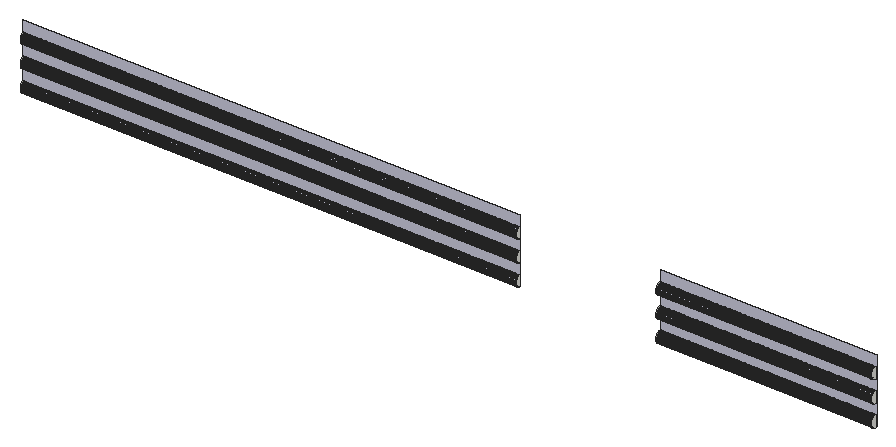
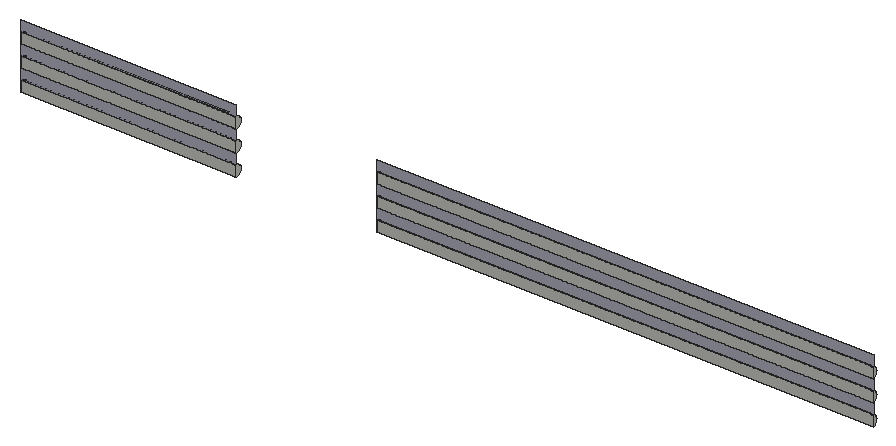
# SketchUp Ruby script. Lengths in millimetres.
U = 1.mm
M = Sketchup.active_model
def pt(a) = Geom::Point3d.new(a.map { |v| v * U })
def face(e, loops, mat)
  f = e.add_face(loops[0].map { |a| pt(a) })
  loops[1..].each { |l| e.add_face(l.map { |a| pt(a) }).erase! }
  f.material = f.back_material = mat if mat
  f
end
# faces: each face lists its corners as indices into pts; further lists are holes
def faces(e, pts, list, mat = nil) = list.each { |f| face(e, (f[0].is_a?(Array) ? f : [f]).map { |l| l.map { |i| pts[i] } }, mat) }
# xy, xz, yz: faces in a plane at the given z, y or x. An outline is a flat list of corners, or four numbers for a rectangle; further outlines are holes
def ring(l) = l.size == 4 ? [[l[0], l[1]], [l[2], l[1]], [l[2], l[3]], [l[0], l[3]]] : l.each_slice(2).to_a
def flat(e, list, mat, &to3) = list.each { |f| face(e, (f[0].is_a?(Array) ? f : [f]).map { |l| ring(l).map { |u, v| to3.(u, v) } }, mat) }
def xy(e, z, list, mat = nil) = flat(e, list, mat) { |x, y| [x, y, z] }
def xz(e, y, list, mat = nil) = flat(e, list, mat) { |x, z| [x, y, z] }
def yz(e, x, list, mat = nil) = flat(e, list, mat) { |y, z| [x, y, z] }
def lines(e, pts, list) = list.each { |a, b| e.add_line(pt(pts[a]), pt(pts[b])) }
# prism: a flat outline (further loops are holes) pulled along v
def prism(e, loops, v, mat = nil)
  f = face(e, loops, mat); d = Geom::Vector3d.new(v.map { |x| x * U })
  f.pushpull(f.normal.samedirection?(d) ? d.length : -d.length)
end
def box(e, o, s, mat = nil) = prism(e, [[o, [o[0] + s[0], o[1], o[2]], [o[0] + s[0], o[1] + s[1], o[2]], [o[0], o[1] + s[1], o[2]]]], [0, 0, s[2]], mat)
def at(x, y, z, deg = 0) = Geom::Transformation.translation(pt([x, y, z])) * Geom::Transformation.rotation(ORIGIN, Z_AXIS, deg.degrees)
def axes(o, x, y, z) = Geom::Transformation.new([*x, 0, *y, 0, *z, 0, *pt(o).to_a, 1])
def part(name) = M.definitions.add(name)
# library, detail: a bought-in or finely detailed component or shape, given as its bounding box
def library(name, o, s) = part(name).tap { |d| box(d.entities, o, s) }
def detail(e, o, s) = box(e.add_group.entities, o, s)
def put(e, d, t, mat = nil) = e.add_instance(d, t).tap { |i| i.material = mat if mat }
def group(e, t, mat = nil) = e.add_group.tap { |g| g.transformation = t; g.material = mat if mat }.entities
root = M.entities
M.materials.add("[0116_Lavender]").color = [197, 197, 214]
xz(root,16548.1,[[11038.5,12969.9,25059.3,13274.7],[29021.7,12969.9,35117.7,13274.7],[11038.5,13579.5,25059.3,13884.3],[29021.7,13579.5,35117.7,13884.3],[11038.5,14189.1,25059.3,14493.9],
  [29021.7,14189.1,35117.7,14493.9]])
xz(root,16548.1,[[11038.5,13274.7,25059.3,13579.5],[29021.7,13274.7,35117.7,13579.5],[11038.5,13884.3,25059.3,14189.1],[29021.7,13884.3,35117.7,14189.1],[11038.5,14493.9,25059.3,14798.7],
  [29021.7,14493.9,35117.7,14798.7]],"[0116_Lavender]")
yz(root,11038.5,[[16548.1,12969.9,16536.2,12975.2,16524.8,12981.5,16514,12988.6,16503.7,12996.6,16494.1,13005.4,16485.2,13014.9,16477.1,13025,16469.8,13035.8,16463.4,13047.1,16458,13058.9,16453.4,13071.1,16449.9,13083.6,16447.3,13096.4,16445.8,13109.3,16445.3,13122.3,16445.8,13135.3,16447.3,13148.2,16449.9,13160.9,16453.4,13173.4,16458,13185.6,16463.4,13197.4,16469.8,13208.7,16477.1,13219.5,16485.2,13229.7,16494.1,13239.2,16503.7,13248,16514,13255.9,16524.8,13263.1,16536.2,13269.3,16548.1,13274.7],[16548.1,13579.5,16536.2,13584.8,16524.8,13591.1,16514,13598.2,16503.7,13606.2,16494.1,13615,16485.2,13624.5,16477.1,13634.6,16469.8,13645.4,16463.4,13656.7,16458,13668.5,16453.4,13680.7,16449.9,13693.2,16447.3,13706,16445.8,13718.9,16445.3,13731.9,16445.8,13744.9,16447.3,13757.8,16449.9,13770.5,16453.4,13783,16458,13795.2,16463.4,13807,16469.8,13818.3,16477.1,13829.1,16485.2,13839.3,16494.1,13848.8,16503.7,13857.6,16514,13865.5,16524.8,13872.7,16536.2,13878.9,16548.1,13884.3],[16548.1,14189.1,16536.2,14194.4,16524.8,14200.7,16514,14207.8,16503.7,14215.8,16494.1,14224.6,16485.2,14234.1,16477.1,14244.2,16469.8,14255,16463.4,14266.3,16458,14278.1,16453.4,14290.3,16449.9,14302.8,16447.3,14315.6,16445.8,14328.5,16445.3,14341.5,16445.8,14354.5,16447.3,14367.4,16449.9,14380.1,16453.4,14392.6,16458,14404.8,16463.4,14416.6,16469.8,14427.9,16477.1,14438.7,16485.2,14448.9,16494.1,14458.4,16503.7,14467.2,16514,14475.1,16524.8,14482.3,16536.2,14488.5,16548.1,14493.9]])
yz(root,25059.3,[[16548.1,12969.9,16548.1,13274.7,16536.2,13269.3,16524.8,13263.1,16514,13255.9,16503.7,13248,16494.1,13239.2,16485.2,13229.7,16477.1,13219.5,16469.8,13208.7,16463.4,13197.4,16458,13185.6,16453.4,13173.4,16449.9,13160.9,16447.3,13148.2,16445.8,13135.3,16445.3,13122.3,16445.8,13109.3,16447.3,13096.4,16449.9,13083.6,16453.4,13071.1,16458,13058.9,16463.4,13047.1,16469.8,13035.8,16477.1,13025,16485.2,13014.9,16494.1,13005.4,16503.7,12996.6,16514,12988.6,16524.8,12981.5,16536.2,12975.2],[16548.1,13579.5,16548.1,13884.3,16536.2,13878.9,16524.8,13872.7,16514,13865.5,16503.7,13857.6,16494.1,13848.8,16485.2,13839.3,16477.1,13829.1,16469.8,13818.3,16463.4,13807,16458,13795.2,16453.4,13783,16449.9,13770.5,16447.3,13757.8,16445.8,13744.9,16445.3,13731.9,16445.8,13718.9,16447.3,13706,16449.9,13693.2,16453.4,13680.7,16458,13668.5,16463.4,13656.7,16469.8,13645.4,16477.1,13634.6,16485.2,13624.5,16494.1,13615,16503.7,13606.2,16514,13598.2,16524.8,13591.1,16536.2,13584.8],[16548.1,14189.1,16548.1,14493.9,16536.2,14488.5,16524.8,14482.3,16514,14475.1,16503.7,14467.2,16494.1,14458.4,16485.2,14448.9,16477.1,14438.7,16469.8,14427.9,16463.4,14416.6,16458,14404.8,16453.4,14392.6,16449.9,14380.1,16447.3,14367.4,16445.8,14354.5,16445.3,14341.5,16445.8,14328.5,16447.3,14315.6,16449.9,14302.8,16453.4,14290.3,16458,14278.1,16463.4,14266.3,16469.8,14255,16477.1,14244.2,16485.2,14234.1,16494.1,14224.6,16503.7,14215.8,16514,14207.8,16524.8,14200.7,16536.2,14194.4]])
yz(root,29021.7,[[16548.1,12969.9,16540.1,12970.1,16532.2,12970.7,16524.3,12971.8,16516.4,12973.2,16508.7,12975.1,16501,12977.3,16493.5,12980,16486.1,12983.1,16478.9,12986.5,16471.9,12990.3,16465.1,12994.5,16458.5,12999,16452.2,13003.8,16446.1,13009,16440.3,13014.5,16434.8,13020.3,16429.7,13026.4,16424.8,13032.7,16420.3,13039.3,16416.1,13046.1,16412.3,13053.1,16408.9,13060.3,16405.8,13067.7,16403.2,13075.2,16400.9,13082.8,16399,13090.6,16397.6,13098.4,16396.5,13106.3,16395.9,13114.3,16395.7,13122.3,16395.9,13130.3,16396.5,13138.2,16397.6,13146.1,16399,13154,16400.9,13161.7,16403.2,13169.4,16405.8,13176.9,16408.9,13184.3,16412.3,13191.5,16416.1,13198.5,16420.3,13205.3,16424.8,13211.9,16429.7,13218.2,16434.8,13224.3,16440.3,13230,16446.1,13235.5,16452.2,13240.7,16458.5,13245.6,16465.1,13250.1,16471.9,13254.3,16478.9,13258.1,16486.1,13261.5,16493.5,13264.6,16501,13267.2,16508.7,13269.5,16516.4,13271.3,16524.3,13272.8,16532.2,13273.8,16540.1,13274.5,16548.1,13274.7],[16548.1,13579.5,16540.1,13579.7,16532.2,13580.3,16524.3,13581.4,16516.4,13582.8,16508.7,13584.7,16501,13586.9,16493.5,13589.6,16486.1,13592.7,16478.9,13596.1,16471.9,13599.9,16465.1,13604.1,16458.5,13608.6,16452.2,13613.4,16446.1,13618.6,16440.3,13624.1,16434.8,13629.9,16429.7,13636,16424.8,13642.3,16420.3,13648.9,16416.1,13655.7,16412.3,13662.7,16408.9,13669.9,16405.8,13677.3,16403.2,13684.8,16400.9,13692.4,16399,13700.2,16397.6,13708,16396.5,13715.9,16395.9,13723.9,16395.7,13731.9,16395.9,13739.9,16396.5,13747.8,16397.6,13755.7,16399,13763.6,16400.9,13771.3,16403.2,13779,16405.8,13786.5,16408.9,13793.9,16412.3,13801.1,16416.1,13808.1,16420.3,13814.9,16424.8,13821.5,16429.7,13827.8,16434.8,13833.9,16440.3,13839.6,16446.1,13845.1,16452.2,13850.3,16458.5,13855.2,16465.1,13859.7,16471.9,13863.9,16478.9,13867.7,16486.1,13871.1,16493.5,13874.2,16501,13876.8,16508.7,13879.1,16516.4,13880.9,16524.3,13882.4,16532.2,13883.4,16540.1,13884.1,16548.1,13884.3],[16548.1,14189.1,16540.1,14189.3,16532.2,14189.9,16524.3,14191,16516.4,14192.4,16508.7,14194.3,16501,14196.5,16493.5,14199.2,16486.1,14202.3,16478.9,14205.7,16471.9,14209.5,16465.1,14213.7,16458.5,14218.2,16452.2,14223,16446.1,14228.2,16440.3,14233.7,16434.8,14239.5,16429.7,14245.6,16424.8,14251.9,16420.3,14258.5,16416.1,14265.3,16412.3,14272.3,16408.9,14279.5,16405.8,14286.9,16403.2,14294.4,16400.9,14302,16399,14309.8,16397.6,14317.6,16396.5,14325.5,16395.9,14333.5,16395.7,14341.5,16395.9,14349.5,16396.5,14357.4,16397.6,14365.3,16399,14373.2,16400.9,14380.9,16403.2,14388.6,16405.8,14396.1,16408.9,14403.5,16412.3,14410.7,16416.1,14417.7,16420.3,14424.5,16424.8,14431.1,16429.7,14437.4,16434.8,14443.5,16440.3,14449.2,16446.1,14454.7,16452.2,14459.9,16458.5,14464.8,16465.1,14469.3,16471.9,14473.5,16478.9,14477.3,16486.1,14480.7,16493.5,14483.8,16501,14486.4,16508.7,14488.7,16516.4,14490.5,16524.3,14492,16532.2,14493,16540.1,14493.7,16548.1,14493.9]])
yz(root,35117.7,[[16548.1,12969.9,16548.1,13274.7,16540.1,13274.5,16532.2,13273.8,16524.3,13272.8,16516.4,13271.3,16508.7,13269.5,16501,13267.2,16493.5,13264.6,16486.1,13261.5,16478.9,13258.1,16471.9,13254.3,16465.1,13250.1,16458.5,13245.6,16452.2,13240.7,16446.1,13235.5,16440.3,13230,16434.8,13224.3,16429.7,13218.2,16424.8,13211.9,16420.3,13205.3,16416.1,13198.5,16412.3,13191.5,16408.9,13184.3,16405.8,13176.9,16403.2,13169.4,16400.9,13161.7,16399,13154,16397.6,13146.1,16396.5,13138.2,16395.9,13130.3,16395.7,13122.3,16395.9,13114.3,16396.5,13106.3,16397.6,13098.4,16399,13090.6,16400.9,13082.8,16403.2,13075.2,16405.8,13067.7,16408.9,13060.3,16412.3,13053.1,16416.1,13046.1,16420.3,13039.3,16424.8,13032.7,16429.7,13026.4,16434.8,13020.3,16440.3,13014.5,16446.1,13009,16452.2,13003.8,16458.5,12999,16465.1,12994.5,16471.9,12990.3,16478.9,12986.5,16486.1,12983.1,16493.5,12980,16501,12977.3,16508.7,12975.1,16516.4,12973.2,16524.3,12971.8,16532.2,12970.7,16540.1,12970.1],[16548.1,13579.5,16548.1,13884.3,16540.1,13884.1,16532.2,13883.4,16524.3,13882.4,16516.4,13880.9,16508.7,13879.1,16501,13876.8,16493.5,13874.2,16486.1,13871.1,16478.9,13867.7,16471.9,13863.9,16465.1,13859.7,16458.5,13855.2,16452.2,13850.3,16446.1,13845.1,16440.3,13839.6,16434.8,13833.9,16429.7,13827.8,16424.8,13821.5,16420.3,13814.9,16416.1,13808.1,16412.3,13801.1,16408.9,13793.9,16405.8,13786.5,16403.2,13779,16400.9,13771.3,16399,13763.6,16397.6,13755.7,16396.5,13747.8,16395.9,13739.9,16395.7,13731.9,16395.9,13723.9,16396.5,13715.9,16397.6,13708,16399,13700.2,16400.9,13692.4,16403.2,13684.8,16405.8,13677.3,16408.9,13669.9,16412.3,13662.7,16416.1,13655.7,16420.3,13648.9,16424.8,13642.3,16429.7,13636,16434.8,13629.9,16440.3,13624.1,16446.1,13618.6,16452.2,13613.4,16458.5,13608.6,16465.1,13604.1,16471.9,13599.9,16478.9,13596.1,16486.1,13592.7,16493.5,13589.6,16501,13586.9,16508.7,13584.7,16516.4,13582.8,16524.3,13581.4,16532.2,13580.3,16540.1,13579.7],[16548.1,14189.1,16548.1,14493.9,16540.1,14493.7,16532.2,14493,16524.3,14492,16516.4,14490.5,16508.7,14488.7,16501,14486.4,16493.5,14483.8,16486.1,14480.7,16478.9,14477.3,16471.9,14473.5,16465.1,14469.3,16458.5,14464.8,16452.2,14459.9,16446.1,14454.7,16440.3,14449.2,16434.8,14443.5,16429.7,14437.4,16424.8,14431.1,16420.3,14424.5,16416.1,14417.7,16412.3,14410.7,16408.9,14403.5,16405.8,14396.1,16403.2,14388.6,16400.9,14380.9,16399,14373.2,16397.6,14365.3,16396.5,14357.4,16395.9,14349.5,16395.7,14341.5,16395.9,14333.5,16396.5,14325.5,16397.6,14317.6,16399,14309.8,16400.9,14302,16403.2,14294.4,16405.8,14286.9,16408.9,14279.5,16412.3,14272.3,16416.1,14265.3,16420.3,14258.5,16424.8,14251.9,16429.7,14245.6,16434.8,14239.5,16440.3,14233.7,16446.1,14228.2,16452.2,14223,16458.5,14218.2,16465.1,14213.7,16471.9,14209.5,16478.9,14205.7,16486.1,14202.3,16493.5,14199.2,16501,14196.5,16508.7,14194.3,16516.4,14192.4,16524.3,14191,16532.2,14189.9,16540.1,14189.3]])
p = [[25059.3,16548.1,12969.9],[25059.3,16536.2,12975.2],[11038.5,16536.2,12975.2],[11038.5,16548.1,12969.9],[35117.7,16548.1,12969.9],[35117.7,16540.1,12970.1],
  [29021.7,16540.1,12970.1],[29021.7,16548.1,12969.9],[35117.7,16532.2,12970.7],[29021.7,16532.2,12970.7],[35117.7,16524.3,12971.8],[29021.7,16524.3,12971.8],
  [35117.7,16516.4,12973.2],[29021.7,16516.4,12973.2],[35117.7,16508.7,12975.1],[29021.7,16508.7,12975.1],[35117.7,16501,12977.3],[29021.7,16501,12977.3],
  [25059.3,16524.8,12981.5],[11038.5,16524.8,12981.5],[35117.7,16493.5,12980],[29021.7,16493.5,12980],[35117.7,16486.1,12983.1],[29021.7,16486.1,12983.1],
  [25059.3,16514,12988.6],[11038.5,16514,12988.6],[35117.7,16478.9,12986.5],[29021.7,16478.9,12986.5],[35117.7,16471.9,12990.3],[29021.7,16471.9,12990.3],
  [25059.3,16503.7,12996.6],[11038.5,16503.7,12996.6],[35117.7,16465.1,12994.5],[29021.7,16465.1,12994.5],[35117.7,16458.5,12999],[29021.7,16458.5,12999],
  [25059.3,16494.1,13005.4],[11038.5,16494.1,13005.4],[35117.7,16452.2,13003.8],[29021.7,16452.2,13003.8],[35117.7,16446.1,13009],[29021.7,16446.1,13009],
  [25059.3,16485.2,13014.9],[11038.5,16485.2,13014.9],[35117.7,16440.3,13014.5],[29021.7,16440.3,13014.5],[35117.7,16434.8,13020.3],[29021.7,16434.8,13020.3],
  [25059.3,16477.1,13025],[11038.5,16477.1,13025],[35117.7,16429.7,13026.4],[29021.7,16429.7,13026.4],[25059.3,16469.8,13035.8],[11038.5,16469.8,13035.8],
  [35117.7,16424.8,13032.7],[29021.7,16424.8,13032.7],[35117.7,16420.3,13039.3],[29021.7,16420.3,13039.3],[25059.3,16463.4,13047.1],[11038.5,16463.4,13047.1],
  [35117.7,16416.1,13046.1],[29021.7,16416.1,13046.1],[35117.7,16412.3,13053.1],[29021.7,16412.3,13053.1],[25059.3,16458,13058.9],[11038.5,16458,13058.9],
  [35117.7,16408.9,13060.3],[29021.7,16408.9,13060.3],[25059.3,16453.4,13071.1],[11038.5,16453.4,13071.1],[35117.7,16405.8,13067.7],[29021.7,16405.8,13067.7],
  [35117.7,16403.2,13075.2],[29021.7,16403.2,13075.2],[25059.3,16449.9,13083.6],[11038.5,16449.9,13083.6],[35117.7,16400.9,13082.8],[29021.7,16400.9,13082.8],
  [35117.7,16399,13090.6],[29021.7,16399,13090.6],[25059.3,16447.3,13096.4],[11038.5,16447.3,13096.4],[35117.7,16397.6,13098.4],[29021.7,16397.6,13098.4],
  [25059.3,16445.8,13109.3],[11038.5,16445.8,13109.3],[35117.7,16396.5,13106.3],[29021.7,16396.5,13106.3],[35117.7,16395.9,13114.3],[29021.7,16395.9,13114.3],
  [25059.3,16445.3,13122.3],[11038.5,16445.3,13122.3],[35117.7,16395.7,13122.3],[29021.7,16395.7,13122.3],[35117.7,16395.9,13130.3],[29021.7,16395.9,13130.3],
  [25059.3,16445.8,13135.3],[11038.5,16445.8,13135.3],[35117.7,16396.5,13138.2],[29021.7,16396.5,13138.2],[25059.3,16447.3,13148.2],[11038.5,16447.3,13148.2],
  [35117.7,16397.6,13146.1],[29021.7,16397.6,13146.1],[35117.7,16399,13154],[29021.7,16399,13154],[25059.3,16449.9,13160.9],[11038.5,16449.9,13160.9],
  [35117.7,16400.9,13161.7],[29021.7,16400.9,13161.7],[25059.3,16453.4,13173.4],[11038.5,16453.4,13173.4],[35117.7,16403.2,13169.4],[29021.7,16403.2,13169.4],
  [35117.7,16405.8,13176.9],[29021.7,16405.8,13176.9],[25059.3,16458,13185.6],[11038.5,16458,13185.6],[35117.7,16408.9,13184.3],[29021.7,16408.9,13184.3],
  [35117.7,16412.3,13191.5],[29021.7,16412.3,13191.5],[25059.3,16463.4,13197.4],[11038.5,16463.4,13197.4],[35117.7,16416.1,13198.5],[29021.7,16416.1,13198.5],
  [25059.3,16469.8,13208.7],[11038.5,16469.8,13208.7],[35117.7,16420.3,13205.3],[29021.7,16420.3,13205.3],[35117.7,16424.8,13211.9],[29021.7,16424.8,13211.9],
  [25059.3,16477.1,13219.5],[11038.5,16477.1,13219.5],[35117.7,16429.7,13218.2],[29021.7,16429.7,13218.2],[35117.7,16434.8,13224.3],[29021.7,16434.8,13224.3],
  [25059.3,16485.2,13229.7],[11038.5,16485.2,13229.7],[35117.7,16440.3,13230],[29021.7,16440.3,13230],[25059.3,16494.1,13239.2],[11038.5,16494.1,13239.2],
  [35117.7,16446.1,13235.5],[29021.7,16446.1,13235.5],[35117.7,16452.2,13240.7],[29021.7,16452.2,13240.7],[25059.3,16503.7,13248],[11038.5,16503.7,13248],
  [35117.7,16458.5,13245.6],[29021.7,16458.5,13245.6],[35117.7,16465.1,13250.1],[29021.7,16465.1,13250.1],[25059.3,16514,13255.9],[11038.5,16514,13255.9],
  [35117.7,16471.9,13254.3],[29021.7,16471.9,13254.3],[35117.7,16478.9,13258.1],[29021.7,16478.9,13258.1],[25059.3,16524.8,13263.1],[11038.5,16524.8,13263.1],
  [35117.7,16486.1,13261.5],[29021.7,16486.1,13261.5],[35117.7,16493.5,13264.6],[29021.7,16493.5,13264.6],[25059.3,16536.2,13269.3],[11038.5,16536.2,13269.3],
  [35117.7,16501,13267.2],[29021.7,16501,13267.2],[35117.7,16508.7,13269.5],[29021.7,16508.7,13269.5],[25059.3,16548.1,13274.7],[11038.5,16548.1,13274.7],
  [35117.7,16516.4,13271.3],[29021.7,16516.4,13271.3],[35117.7,16524.3,13272.8],[29021.7,16524.3,13272.8],[35117.7,16532.2,13273.8],[29021.7,16532.2,13273.8],
  [35117.7,16540.1,13274.5],[29021.7,16540.1,13274.5],[35117.7,16548.1,13274.7],[29021.7,16548.1,13274.7],[25059.3,16548.1,13579.5],[25059.3,16536.2,13584.8],
  [11038.5,16536.2,13584.8],[11038.5,16548.1,13579.5],[35117.7,16548.1,13579.5],[35117.7,16540.1,13579.7],[29021.7,16540.1,13579.7],[29021.7,16548.1,13579.5],
  [35117.7,16532.2,13580.3],[29021.7,16532.2,13580.3],[35117.7,16524.3,13581.4],[29021.7,16524.3,13581.4],[35117.7,16516.4,13582.8],[29021.7,16516.4,13582.8],
  [35117.7,16508.7,13584.7],[29021.7,16508.7,13584.7],[35117.7,16501,13586.9],[29021.7,16501,13586.9],[25059.3,16524.8,13591.1],[11038.5,16524.8,13591.1],
  [35117.7,16493.5,13589.6],[29021.7,16493.5,13589.6],[35117.7,16486.1,13592.7],[29021.7,16486.1,13592.7],[25059.3,16514,13598.2],[11038.5,16514,13598.2],
  [35117.7,16478.9,13596.1],[29021.7,16478.9,13596.1],[35117.7,16471.9,13599.9],[29021.7,16471.9,13599.9],[25059.3,16503.7,13606.2],[11038.5,16503.7,13606.2],
  [35117.7,16465.1,13604.1],[29021.7,16465.1,13604.1],[35117.7,16458.5,13608.6],[29021.7,16458.5,13608.6],[25059.3,16494.1,13615],[11038.5,16494.1,13615],
  [35117.7,16452.2,13613.4],[29021.7,16452.2,13613.4],[35117.7,16446.1,13618.6],[29021.7,16446.1,13618.6],[25059.3,16485.2,13624.5],[11038.5,16485.2,13624.5],
  [35117.7,16440.3,13624.1],[29021.7,16440.3,13624.1],[35117.7,16434.8,13629.9],[29021.7,16434.8,13629.9],[25059.3,16477.1,13634.6],[11038.5,16477.1,13634.6],
  [35117.7,16429.7,13636],[29021.7,16429.7,13636],[25059.3,16469.8,13645.4],[11038.5,16469.8,13645.4],[35117.7,16424.8,13642.3],[29021.7,16424.8,13642.3],
  [35117.7,16420.3,13648.9],[29021.7,16420.3,13648.9],[25059.3,16463.4,13656.7],[11038.5,16463.4,13656.7],[35117.7,16416.1,13655.7],[29021.7,16416.1,13655.7],
  [35117.7,16412.3,13662.7],[29021.7,16412.3,13662.7],[25059.3,16458,13668.5],[11038.5,16458,13668.5],[35117.7,16408.9,13669.9],[29021.7,16408.9,13669.9],
  [25059.3,16453.4,13680.7],[11038.5,16453.4,13680.7],[35117.7,16405.8,13677.3],[29021.7,16405.8,13677.3],[35117.7,16403.2,13684.8],[29021.7,16403.2,13684.8],
  [25059.3,16449.9,13693.2],[11038.5,16449.9,13693.2],[35117.7,16400.9,13692.4],[29021.7,16400.9,13692.4],[35117.7,16399,13700.2],[29021.7,16399,13700.2],
  [25059.3,16447.3,13706],[11038.5,16447.3,13706],[35117.7,16397.6,13708],[29021.7,16397.6,13708],[25059.3,16445.8,13718.9],[11038.5,16445.8,13718.9],
  [35117.7,16396.5,13715.9],[29021.7,16396.5,13715.9],[35117.7,16395.9,13723.9],[29021.7,16395.9,13723.9],[25059.3,16445.3,13731.9],[11038.5,16445.3,13731.9],
  [35117.7,16395.7,13731.9],[29021.7,16395.7,13731.9],[35117.7,16395.9,13739.9],[29021.7,16395.9,13739.9],[25059.3,16445.8,13744.9],[11038.5,16445.8,13744.9],
  [35117.7,16396.5,13747.8],[29021.7,16396.5,13747.8],[25059.3,16447.3,13757.8],[11038.5,16447.3,13757.8],[35117.7,16397.6,13755.7],[29021.7,16397.6,13755.7],
  [35117.7,16399,13763.6],[29021.7,16399,13763.6],[25059.3,16449.9,13770.5],[11038.5,16449.9,13770.5],[35117.7,16400.9,13771.3],[29021.7,16400.9,13771.3],
  [25059.3,16453.4,13783],[11038.5,16453.4,13783],[35117.7,16403.2,13779],[29021.7,16403.2,13779],[35117.7,16405.8,13786.5],[29021.7,16405.8,13786.5],
  [25059.3,16458,13795.2],[11038.5,16458,13795.2],[35117.7,16408.9,13793.9],[29021.7,16408.9,13793.9],[35117.7,16412.3,13801.1],[29021.7,16412.3,13801.1],
  [25059.3,16463.4,13807],[11038.5,16463.4,13807],[35117.7,16416.1,13808.1],[29021.7,16416.1,13808.1],[25059.3,16469.8,13818.3],[11038.5,16469.8,13818.3],
  [35117.7,16420.3,13814.9],[29021.7,16420.3,13814.9],[35117.7,16424.8,13821.5],[29021.7,16424.8,13821.5],[25059.3,16477.1,13829.1],[11038.5,16477.1,13829.1],
  [35117.7,16429.7,13827.8],[29021.7,16429.7,13827.8],[35117.7,16434.8,13833.9],[29021.7,16434.8,13833.9],[25059.3,16485.2,13839.3],[11038.5,16485.2,13839.3],
  [35117.7,16440.3,13839.6],[29021.7,16440.3,13839.6],[25059.3,16494.1,13848.8],[11038.5,16494.1,13848.8],[35117.7,16446.1,13845.1],[29021.7,16446.1,13845.1],
  [35117.7,16452.2,13850.3],[29021.7,16452.2,13850.3],[25059.3,16503.7,13857.6],[11038.5,16503.7,13857.6],[35117.7,16458.5,13855.2],[29021.7,16458.5,13855.2],
  [35117.7,16465.1,13859.7],[29021.7,16465.1,13859.7],[25059.3,16514,13865.5],[11038.5,16514,13865.5],[35117.7,16471.9,13863.9],[29021.7,16471.9,13863.9],
  [35117.7,16478.9,13867.7],[29021.7,16478.9,13867.7],[25059.3,16524.8,13872.7],[11038.5,16524.8,13872.7],[35117.7,16486.1,13871.1],[29021.7,16486.1,13871.1],
  [35117.7,16493.5,13874.2],[29021.7,16493.5,13874.2],[25059.3,16536.2,13878.9],[11038.5,16536.2,13878.9],[35117.7,16501,13876.8],[29021.7,16501,13876.8],
  [35117.7,16508.7,13879.1],[29021.7,16508.7,13879.1],[25059.3,16548.1,13884.3],[11038.5,16548.1,13884.3],[35117.7,16516.4,13880.9],[29021.7,16516.4,13880.9],
  [35117.7,16524.3,13882.4],[29021.7,16524.3,13882.4],[35117.7,16532.2,13883.4],[29021.7,16532.2,13883.4],[35117.7,16540.1,13884.1],[29021.7,16540.1,13884.1],
  [35117.7,16548.1,13884.3],[29021.7,16548.1,13884.3],[25059.3,16548.1,14189.1],[25059.3,16536.2,14194.4],[11038.5,16536.2,14194.4],[11038.5,16548.1,14189.1],
  [35117.7,16548.1,14189.1],[35117.7,16540.1,14189.3],[29021.7,16540.1,14189.3],[29021.7,16548.1,14189.1],[35117.7,16532.2,14189.9],[29021.7,16532.2,14189.9],
  [35117.7,16524.3,14191],[29021.7,16524.3,14191],[35117.7,16516.4,14192.4],[29021.7,16516.4,14192.4],[35117.7,16508.7,14194.3],[29021.7,16508.7,14194.3],
  [35117.7,16501,14196.5],[29021.7,16501,14196.5],[25059.3,16524.8,14200.7],[11038.5,16524.8,14200.7],[35117.7,16493.5,14199.2],[29021.7,16493.5,14199.2],
  [35117.7,16486.1,14202.3],[29021.7,16486.1,14202.3],[25059.3,16514,14207.8],[11038.5,16514,14207.8],[35117.7,16478.9,14205.7],[29021.7,16478.9,14205.7],
  [35117.7,16471.9,14209.5],[29021.7,16471.9,14209.5],[25059.3,16503.7,14215.8],[11038.5,16503.7,14215.8],[35117.7,16465.1,14213.7],[29021.7,16465.1,14213.7],
  [35117.7,16458.5,14218.2],[29021.7,16458.5,14218.2],[25059.3,16494.1,14224.6],[11038.5,16494.1,14224.6],[35117.7,16452.2,14223],[29021.7,16452.2,14223],
  [35117.7,16446.1,14228.2],[29021.7,16446.1,14228.2],[25059.3,16485.2,14234.1],[11038.5,16485.2,14234.1],[35117.7,16440.3,14233.7],[29021.7,16440.3,14233.7],
  [35117.7,16434.8,14239.5],[29021.7,16434.8,14239.5],[25059.3,16477.1,14244.2],[11038.5,16477.1,14244.2],[35117.7,16429.7,14245.6],[29021.7,16429.7,14245.6],
  [25059.3,16469.8,14255],[11038.5,16469.8,14255],[35117.7,16424.8,14251.9],[29021.7,16424.8,14251.9],[35117.7,16420.3,14258.5],[29021.7,16420.3,14258.5],
  [25059.3,16463.4,14266.3],[11038.5,16463.4,14266.3],[35117.7,16416.1,14265.3],[29021.7,16416.1,14265.3],[35117.7,16412.3,14272.3],[29021.7,16412.3,14272.3],
  [25059.3,16458,14278.1],[11038.5,16458,14278.1],[35117.7,16408.9,14279.5],[29021.7,16408.9,14279.5],[25059.3,16453.4,14290.3],[11038.5,16453.4,14290.3],
  [35117.7,16405.8,14286.9],[29021.7,16405.8,14286.9],[35117.7,16403.2,14294.4],[29021.7,16403.2,14294.4],[25059.3,16449.9,14302.8],[11038.5,16449.9,14302.8],
  [35117.7,16400.9,14302],[29021.7,16400.9,14302],[35117.7,16399,14309.8],[29021.7,16399,14309.8],[25059.3,16447.3,14315.6],[11038.5,16447.3,14315.6],
  [35117.7,16397.6,14317.6],[29021.7,16397.6,14317.6],[25059.3,16445.8,14328.5],[11038.5,16445.8,14328.5],[35117.7,16396.5,14325.5],[29021.7,16396.5,14325.5],
  [35117.7,16395.9,14333.5],[29021.7,16395.9,14333.5],[25059.3,16445.3,14341.5],[11038.5,16445.3,14341.5],[35117.7,16395.7,14341.5],[29021.7,16395.7,14341.5],
  [35117.7,16395.9,14349.5],[29021.7,16395.9,14349.5],[25059.3,16445.8,14354.5],[11038.5,16445.8,14354.5],[35117.7,16396.5,14357.4],[29021.7,16396.5,14357.4],
  [25059.3,16447.3,14367.4],[11038.5,16447.3,14367.4],[35117.7,16397.6,14365.3],[29021.7,16397.6,14365.3],[35117.7,16399,14373.2],[29021.7,16399,14373.2],
  [25059.3,16449.9,14380.1],[11038.5,16449.9,14380.1],[35117.7,16400.9,14380.9],[29021.7,16400.9,14380.9],[25059.3,16453.4,14392.6],[11038.5,16453.4,14392.6],
  [35117.7,16403.2,14388.6],[29021.7,16403.2,14388.6],[35117.7,16405.8,14396.1],[29021.7,16405.8,14396.1],[25059.3,16458,14404.8],[11038.5,16458,14404.8],
  [35117.7,16408.9,14403.5],[29021.7,16408.9,14403.5],[35117.7,16412.3,14410.7],[29021.7,16412.3,14410.7],[25059.3,16463.4,14416.6],[11038.5,16463.4,14416.6],
  [35117.7,16416.1,14417.7],[29021.7,16416.1,14417.7],[25059.3,16469.8,14427.9],[11038.5,16469.8,14427.9],[35117.7,16420.3,14424.5],[29021.7,16420.3,14424.5],
  [35117.7,16424.8,14431.1],[29021.7,16424.8,14431.1],[25059.3,16477.1,14438.7],[11038.5,16477.1,14438.7],[35117.7,16429.7,14437.4],[29021.7,16429.7,14437.4],
  [35117.7,16434.8,14443.5],[29021.7,16434.8,14443.5],[25059.3,16485.2,14448.9],[11038.5,16485.2,14448.9],[35117.7,16440.3,14449.2],[29021.7,16440.3,14449.2],
  [25059.3,16494.1,14458.4],[11038.5,16494.1,14458.4],[35117.7,16446.1,14454.7],[29021.7,16446.1,14454.7],[35117.7,16452.2,14459.9],[29021.7,16452.2,14459.9],
  [25059.3,16503.7,14467.2],[11038.5,16503.7,14467.2],[35117.7,16458.5,14464.8],[29021.7,16458.5,14464.8],[35117.7,16465.1,14469.3],[29021.7,16465.1,14469.3],
  [25059.3,16514,14475.1],[11038.5,16514,14475.1],[35117.7,16471.9,14473.5],[29021.7,16471.9,14473.5],[35117.7,16478.9,14477.3],[29021.7,16478.9,14477.3],
  [25059.3,16524.8,14482.3],[11038.5,16524.8,14482.3],[35117.7,16486.1,14480.7],[29021.7,16486.1,14480.7],[35117.7,16493.5,14483.8],[29021.7,16493.5,14483.8],
  [25059.3,16536.2,14488.5],[11038.5,16536.2,14488.5],[35117.7,16501,14486.4],[29021.7,16501,14486.4],[35117.7,16508.7,14488.7],[29021.7,16508.7,14488.7],
  [25059.3,16548.1,14493.9],[11038.5,16548.1,14493.9],[35117.7,16516.4,14490.5],[29021.7,16516.4,14490.5],[35117.7,16524.3,14492],[29021.7,16524.3,14492],
  [35117.7,16532.2,14493],[29021.7,16532.2,14493],[35117.7,16540.1,14493.7],[29021.7,16540.1,14493.7],[35117.7,16548.1,14493.9],[29021.7,16548.1,14493.9]]
faces(root,p,[[0,1,2,3],[4,5,6,7],[5,8,9,6],[8,10,11,9],[10,12,13,11],[12,14,15,13],[14,16,17,15],[1,18,19,2],
  [16,20,21,17],[20,22,23,21],[18,24,25,19],[22,26,27,23],[26,28,29,27],[24,30,31,25],[28,32,33,29],[32,34,35,33],
  [30,36,37,31],[34,38,39,35],[38,40,41,39],[36,42,43,37],[40,44,45,41],[44,46,47,45],[42,48,49,43],[46,50,51,47],
  [48,52,53,49],[50,54,55,51],[54,56,57,55],[52,58,59,53],[56,60,61,57],[60,62,63,61],[58,64,65,59],[62,66,67,63],
  [64,68,69,65],[66,70,71,67],[70,72,73,71],[68,74,75,69],[72,76,77,73],[76,78,79,77],[74,80,81,75],[78,82,83,79],
  [80,84,85,81],[82,86,87,83],[86,88,89,87],[84,90,91,85],[88,92,93,89],[92,94,95,93],[90,96,97,91],[94,98,99,95],
  [96,100,101,97],[98,102,103,99],[102,104,105,103],[100,106,107,101],[104,108,109,105],[106,110,111,107],[108,112,113,109],[112,114,115,113],
  [110,116,117,111],[114,118,119,115],[118,120,121,119],[116,122,123,117],[120,124,125,121],[122,126,127,123],[124,128,129,125],[128,130,131,129],
  [126,132,133,127],[130,134,135,131],[134,136,137,135],[132,138,139,133],[136,140,141,137],[138,142,143,139],[140,144,145,141],[144,146,147,145],
  [142,148,149,143],[146,150,151,147],[150,152,153,151],[148,154,155,149],[152,156,157,153],[156,158,159,157],[154,160,161,155],[158,162,163,159],
  [162,164,165,163],[160,166,167,161],[164,168,169,165],[168,170,171,169],[166,172,173,167],[170,174,175,171],[174,176,177,175],[176,178,179,177],
  [178,180,181,179],[180,182,183,181],[184,185,186,187],[188,189,190,191],[189,192,193,190],[192,194,195,193],[194,196,197,195],[196,198,199,197],
  [198,200,201,199],[185,202,203,186],[200,204,205,201],[204,206,207,205],[202,208,209,203],[206,210,211,207],[210,212,213,211],[208,214,215,209],
  [212,216,217,213],[216,218,219,217],[214,220,221,215],[218,222,223,219],[222,224,225,223],[220,226,227,221],[224,228,229,225],[228,230,231,229],
  [226,232,233,227],[230,234,235,231],[232,236,237,233],[234,238,239,235],[238,240,241,239],[236,242,243,237],[240,244,245,241],[244,246,247,245],
  [242,248,249,243],[246,250,251,247],[248,252,253,249],[250,254,255,251],[254,256,257,255],[252,258,259,253],[256,260,261,257],[260,262,263,261],
  [258,264,265,259],[262,266,267,263],[264,268,269,265],[266,270,271,267],[270,272,273,271],[268,274,275,269],[272,276,277,273],[276,278,279,277],
  [274,280,281,275],[278,282,283,279],[280,284,285,281],[282,286,287,283],[286,288,289,287],[284,290,291,285],[288,292,293,289],[290,294,295,291],
  [292,296,297,293],[296,298,299,297],[294,300,301,295],[298,302,303,299],[302,304,305,303],[300,306,307,301],[304,308,309,305],[306,310,311,307],
  [308,312,313,309],[312,314,315,313],[310,316,317,311],[314,318,319,315],[318,320,321,319],[316,322,323,317],[320,324,325,321],[322,326,327,323],
  [324,328,329,325],[328,330,331,329],[326,332,333,327],[330,334,335,331],[334,336,337,335],[332,338,339,333],[336,340,341,337],[340,342,343,341],
  [338,344,345,339],[342,346,347,343],[346,348,349,347],[344,350,351,345],[348,352,353,349],[352,354,355,353],[350,356,357,351],[354,358,359,355],
  [358,360,361,359],[360,362,363,361],[362,364,365,363],[364,366,367,365],[368,369,370,371],[372,373,374,375],[373,376,377,374],[376,378,379,377],
  [378,380,381,379],[380,382,383,381],[382,384,385,383],[369,386,387,370],[384,388,389,385],[388,390,391,389],[386,392,393,387],[390,394,395,391],
  [394,396,397,395],[392,398,399,393],[396,400,401,397],[400,402,403,401],[398,404,405,399],[402,406,407,403],[406,408,409,407],[404,410,411,405],
  [408,412,413,409],[412,414,415,413],[410,416,417,411],[414,418,419,415],[416,420,421,417],[418,422,423,419],[422,424,425,423],[420,426,427,421],
  [424,428,429,425],[428,430,431,429],[426,432,433,427],[430,434,435,431],[432,436,437,433],[434,438,439,435],[438,440,441,439],[436,442,443,437],
  [440,444,445,441],[444,446,447,445],[442,448,449,443],[446,450,451,447],[448,452,453,449],[450,454,455,451],[454,456,457,455],[452,458,459,453],
  [456,460,461,457],[460,462,463,461],[458,464,465,459],[462,466,467,463],[464,468,469,465],[466,470,471,467],[470,472,473,471],[468,474,475,469],
  [472,476,477,473],[474,478,479,475],[476,480,481,477],[480,482,483,481],[478,484,485,479],[482,486,487,483],[486,488,489,487],[484,490,491,485],
  [488,492,493,489],[490,494,495,491],[492,496,497,493],[496,498,499,497],[494,500,501,495],[498,502,503,499],[502,504,505,503],[500,506,507,501],
  [504,508,509,505],[506,510,511,507],[508,512,513,509],[512,514,515,513],[510,516,517,511],[514,518,519,515],[518,520,521,519],[516,522,523,517],
  [520,524,525,521],[524,526,527,525],[522,528,529,523],[526,530,531,527],[530,532,533,531],[528,534,535,529],[532,536,537,533],[536,538,539,537],
  [534,540,541,535],[538,542,543,539],[542,544,545,543],[544,546,547,545],[546,548,549,547],[548,550,551,549]],"[0116_Lavender]")
